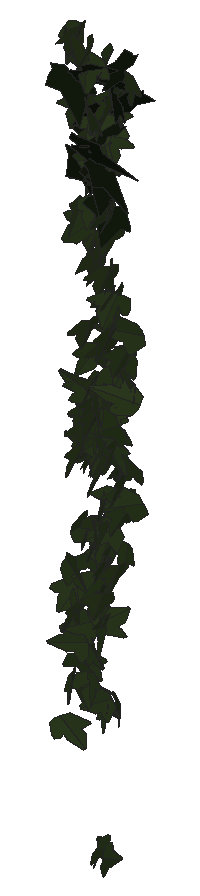
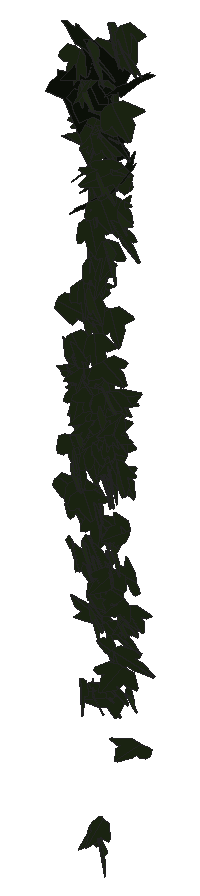
# SketchUp Ruby script. Lengths in inches.
U = 1.inch
M = Sketchup.active_model
def pt(a) = Geom::Point3d.new(a.map { |v| v * U })
def face(e, loops, mat)
  f = e.add_face(loops[0].map { |a| pt(a) })
  loops[1..].each { |l| e.add_face(l.map { |a| pt(a) }).erase! }
  f.material = f.back_material = mat if mat
  f
end
# faces: each face lists its corners as indices into pts; further lists are holes
def faces(e, pts, list, mat = nil) = list.each { |f| face(e, (f[0].is_a?(Array) ? f : [f]).map { |l| l.map { |i| pts[i] } }, mat) }
# xy, xz, yz: faces in a plane at the given z, y or x. An outline is a flat list of corners, or four numbers for a rectangle; further outlines are holes
def ring(l) = l.size == 4 ? [[l[0], l[1]], [l[2], l[1]], [l[2], l[3]], [l[0], l[3]]] : l.each_slice(2).to_a
def flat(e, list, mat, &to3) = list.each { |f| face(e, (f[0].is_a?(Array) ? f : [f]).map { |l| ring(l).map { |u, v| to3.(u, v) } }, mat) }
def xy(e, z, list, mat = nil) = flat(e, list, mat) { |x, y| [x, y, z] }
def xz(e, y, list, mat = nil) = flat(e, list, mat) { |x, z| [x, y, z] }
def yz(e, x, list, mat = nil) = flat(e, list, mat) { |y, z| [x, y, z] }
def lines(e, pts, list) = list.each { |a, b| e.add_line(pt(pts[a]), pt(pts[b])) }
# prism: a flat outline (further loops are holes) pulled along v
def prism(e, loops, v, mat = nil)
  f = face(e, loops, mat); d = Geom::Vector3d.new(v.map { |x| x * U })
  f.pushpull(f.normal.samedirection?(d) ? d.length : -d.length)
end
def box(e, o, s, mat = nil) = prism(e, [[o, [o[0] + s[0], o[1], o[2]], [o[0] + s[0], o[1] + s[1], o[2]], [o[0], o[1] + s[1], o[2]]]], [0, 0, s[2]], mat)
def at(x, y, z, deg = 0) = Geom::Transformation.translation(pt([x, y, z])) * Geom::Transformation.rotation(ORIGIN, Z_AXIS, deg.degrees)
def axes(o, x, y, z) = Geom::Transformation.new([*x, 0, *y, 0, *z, 0, *pt(o).to_a, 1])
def part(name) = M.definitions.add(name)
# library, detail: a bought-in or finely detailed component or shape, given as its bounding box
def library(name, o, s) = part(name).tap { |d| box(d.entities, o, s) }
def detail(e, o, s) = box(e.add_group.entities, o, s)
def put(e, d, t, mat = nil) = e.add_instance(d, t).tap { |i| i.material = mat if mat }
def group(e, t, mat = nil) = e.add_group.tap { |g| g.transformation = t; g.material = mat if mat }.entities
root = M.entities
M.materials.add("1026 AP 7946 SUNNY SIDE UP").color = [254, 231, 186]
M.materials.add("efeu1").color = [18, 25, 13]
M.materials.add("efeu2").color = [43, 57, 29]
c1 = part("ivyleaf_10")
p = [[0,0.5,-0.03],[-0.0625,2.02,-0.43],[-0.19,2.01,-0.46],[-0.54,1.05,-0.29],[-0.52,0.625,-0.18],[-0.83,0.76,-0.28],
  [-1.16,0.64,-0.33],[-1.15,0.33,-0.24],[-0.77,-0.39,0.02],[-0.3,-0.51,0.16],[0.04,-0.48,0.23],[-0.02,2.01,-0.4375],
  [-0.06,2.01,-0.43],[0.04,-0.49,0.23],[0.67,-0.49,0.14],[1.38,0.36,-0.2],[1.375,0.51,-0.24],[0.81,0.65,-0.19],
  [0.62,0.59,-0.15],[0.6,1.09,-0.28],[0.5,1.23,-0.31]]
faces(c1.entities,p,[[0,1,2,3,4,5,6,7,8,9,10],[11,12,0,13,14,15,16,17,18,19,20]],"efeu2")
c2 = part("ivyleaf_9")
p = [[1.54,2.16,1.25],[1.36,2.04,1.19],[-0.21,0.99,0.68],[-0.71,1.11,0.82],[-0.85,0.86,0.67],[-0.8,0.17,0.21],
  [-0.9,-0.01,0.1],[-0.67,-0.16,-0.02],[-0.08,-0.08,-0.05],[-0.03,-0.6,-0.4],[0.65,-0.88,-0.66],[0.83,-0.6,-0.49],
  [1.29,-0.42,-0.43],[1.8125,-0.07,-0.26],[1.21,0.44,0.15]]
faces(c2.entities,p,[[0,1,2,3,4,5,6,7,8,9,10,11,12,13,14]],"efeu1")
put(root,c1,axes([96.59,212.76,256.66],[0.16528,-0.03339,-0.18493],[-0.28245,0.01701,-0.11164],[0.04984,0.20716,-0.01939]),"1026 AP 7946 SUNNY SIDE UP")
put(root,c1,axes([96.42,212.9375,259.95],[0.03193,-0.19079,0.09635],[0.02892,-0.09312,-0.19805],[0.33361,0.02633,0.00795]),"1026 AP 7946 SUNNY SIDE UP")
put(root,c1,axes([96.55,212.97,260.11],[-0.3057,0.02603,0.089],[-0.13977,-0.02208,-0.19969],[-0.02302,-0.21154,0.03053]),"1026 AP 7946 SUNNY SIDE UP")
put(root,c1,axes([96.36,212.93,267.5],[0.28838,-0.15534,0.08831],[0.07617,-0.07607,-0.24669],[0.26908,0.18802,-0.02482]),"1026 AP 7946 SUNNY SIDE UP")
put(root,c1,axes([96.45,212.8,257.53],[0.30391,0.0384,-0.06901],[-0.09836,-0.02901,-0.20255],[-0.0717,0.20256,-0.01467]),"1026 AP 7946 SUNNY SIDE UP")
put(root,c1,axes([96.3125,212.73,255.11],[0.20943,0.10817,0.11767],[0.1516,0.06111,-0.17603],[-0.19457,0.16404,-0.0105]),"1026 AP 7946 SUNNY SIDE UP")
put(root,c1,axes([96.55,212.71,267.67],[-0.02234,-0.25481,-0.00265],[0.00583,0.00092,-0.26288],[0.40063,-0.01422,0.00368]),"1026 AP 7946 SUNNY SIDE UP")
put(root,c1,axes([96.61,212.87,266.35],[-0.1677,-0.21279,0.08333],[-0.02614,-0.08313,-0.24472],[0.35767,-0.10584,0.02118]),"1026 AP 7946 SUNNY SIDE UP")
put(root,c1,axes([96.59,212.95,260.78],[-0.04227,-0.2068,0.07166],[-0.00557,-0.07084,-0.21519],[0.34363,-0.02659,0.00533]),"1026 AP 7946 SUNNY SIDE UP")
put(root,c1,axes([96.59,212.92,260.48],[-0.10699,-0.20863,-0.01607],[0.01691,0.01165,-0.22591],[0.3284,-0.06857,0.00639]),"1026 AP 7946 SUNNY SIDE UP")
put(root,c1,axes([96.56,212.68,257.3],[0.05615,-0.02915,-0.22101],[0.02756,0.21694,-0.02611],[0.33905,-0.01281,0.03872]),"1026 AP 7946 SUNNY SIDE UP")
put(root,c1,axes([96.8,212.81,261.16],[-0.18364,-0.02128,-0.19752],[-0.30314,0.01117,0.11984],[-0.00232,0.22412,-0.0234]),"1026 AP 7946 SUNNY SIDE UP")
put(root,c1,axes([96.45,212.73,255.99],[0.12305,-0.09537,0.17263],[0.15601,-0.13583,-0.12776],[0.26082,0.12624,-0.00503]),"1026 AP 7946 SUNNY SIDE UP")
put(root,c1,axes([96.55,212.63,267.52],[-0.30771,0.1632,-0.02854],[0.00764,-0.0378,-0.26029],[-0.28121,-0.1796,0.02416]),"1026 AP 7946 SUNNY SIDE UP")
put(root,c1,axes([96.59,213,259.97],[0.09491,-0.20168,-0.03352],[-0.00023,0.03269,-0.21648],[0.32095,0.05966,0.00975]),"1026 AP 7946 SUNNY SIDE UP")
put(root,c1,axes([96.59,212.7,257.29],[0.04855,-0.17441,0.10361],[0.01151,-0.10171,-0.18282],[0.31714,0.03039,-0.00923]),"1026 AP 7946 SUNNY SIDE UP")
put(root,c1,axes([96.6875,212.73,264.2],[0.27516,-0.13573,-0.11826],[-0.15734,0.05663,-0.22731],[0.23009,0.20104,-0.01401]),"1026 AP 7946 SUNNY SIDE UP")
put(root,c1,axes([96.73,212.99,260.65],[-0.28813,-0.05134,-0.10827],[-0.1693,-0.00089,0.19439],[-0.0708,0.2111,-0.0242]),"1026 AP 7946 SUNNY SIDE UP")
put(root,c1,axes([96.54,212.99,260.87],[0.01949,0.21668,-0.02469],[-0.00003,-0.02523,-0.22373],[-0.34301,0.01231,-0.00138]),"1026 AP 7946 SUNNY SIDE UP")
put(root,c2,axes([96.49,212.91,265.16],[0.17587,-0.14957,-0.16549],[0.16614,-0.12026,0.19145],[-0.3014,-0.15356,0.00896]),"1026 AP 7946 SUNNY SIDE UP")
put(root,c1,axes([96.75,212.74,257.07],[0.21043,-0.06874,-0.15313],[-0.22571,0.04213,-0.15336],[0.12281,0.19522,-0.01948]),"1026 AP 7946 SUNNY SIDE UP")
put(root,c2,axes([96.48,212.69,266.83],[-0.02459,-0.25041,-0.01019],[0.00763,0.00819,-0.25839],[0.3939,-0.01579,0.00437]),"1026 AP 7946 SUNNY SIDE UP")
put(root,c1,axes([96.63,212.92,258.62],[0.11432,-0.191,-0.02471],[-0.00597,0.02306,-0.21035],[0.30242,0.07266,0.00519]),"1026 AP 7946 SUNNY SIDE UP")
put(root,c1,axes([96.5625,212.76,264.5],[0.08499,-0.1559,0.17875],[0.11831,-0.15789,-0.17036],[0.34827,0.09168,0.01425]),"1026 AP 7946 SUNNY SIDE UP")
put(root,c1,axes([96.71,212.9,261.22],[-0.25836,-0.13814,0.06274],[-0.02668,-0.07367,-0.21694],[0.23638,-0.1593,0.04409]),"1026 AP 7946 SUNNY SIDE UP")
put(root,c1,axes([96.67,213.03,259.88],[0.12107,-0.18948,-0.05398],[-0.00487,0.05395,-0.20967],[0.30864,0.07518,0.01787]),"1026 AP 7946 SUNNY SIDE UP")
put(root,c1,axes([96.56,212.88,257.67],[-0.27039,0.04284,-0.10368],[0.14124,-0.05246,-0.181],[-0.09875,-0.19234,0.02501]),"1026 AP 7946 SUNNY SIDE UP")
put(root,c1,axes([96.72,212.96,261.84],[0.16955,0.15754,-0.11644],[-0.14754,-0.07192,-0.19438],[-0.26773,0.1394,0.03338]),"1026 AP 7946 SUNNY SIDE UP")
put(root,c1,axes([96.43,212.67,258.01],[0.09325,-0.03481,0.22212],[0.31671,-0.07819,-0.07047],[0.13357,0.20971,0.01203]),"1026 AP 7946 SUNNY SIDE UP")
put(root,c1,axes([96.625,212.97,260.16],[0.00381,0.20896,-0.05279],[-0.00198,-0.05241,-0.21559],[-0.33874,0.00266,0.00067]),"1026 AP 7946 SUNNY SIDE UP")
put(root,c1,axes([96.67,212.62,258.76],[0.03395,-0.02797,0.23445],[-0.05757,0.22539,0.03342],[-0.35616,-0.0391,0.01695]),"1026 AP 7946 SUNNY SIDE UP")
put(root,c1,axes([96.62,212.79,256.36],[-0.26873,-0.07694,-0.09459],[0.141,0.02276,-0.19238],[0.12411,-0.19246,0.01375]),"1026 AP 7946 SUNNY SIDE UP")
put(root,c1,axes([96.74,212.9,263.83],[0.12556,-0.21826,-0.05346],[-0.02461,0.04821,-0.23913],[0.35145,0.08135,0.00236]),"1026 AP 7946 SUNNY SIDE UP")
put(root,c1,axes([96.73,212.89,258.39],[0.10867,-0.17815,-0.07354],[-0.01647,0.07119,-0.19583],[0.30074,0.06827,0.01585]),"1026 AP 7946 SUNNY SIDE UP")
put(root,c1,axes([96.72,212.94,261.34],[0.14003,-0.1976,0.05569],[0.01546,-0.05597,-0.22317],[0.32222,0.08856,-0.01349]),"1026 AP 7946 SUNNY SIDE UP")
put(root,c1,axes([96.77,212.93,261],[0.00581,-0.21472,0.0594],[-0.00322,-0.05891,-0.22156],[0.35007,0.00302,-0.00302]),"1026 AP 7946 SUNNY SIDE UP")
put(root,c1,axes([96.64,212.9375,258.13],[-0.15915,-0.12646,-0.13155],[0.17791,0.068,-0.16227],[0.21852,-0.14746,0.0363]),"1026 AP 7946 SUNNY SIDE UP")
put(root,c1,axes([96.77,212.96,260.5],[-0.33745,-0.00833,-0.00268],[0.00752,-0.06006,-0.21274],[0.01145,-0.20605,0.0608]),"1026 AP 7946 SUNNY SIDE UP")
put(root,c1,axes([96.58,212.91,265.33],[-0.18912,-0.09021,-0.20199],[0.27353,0.09136,-0.1531],[0.19964,-0.21063,0.01841]),"1026 AP 7946 SUNNY SIDE UP")
put(root,c1,axes([96.82,212.92,265.19],[0.06552,-0.23859,0.0421],[0.00101,-0.04274,-0.24967],[0.38098,0.04115,-0.00658]),"1026 AP 7946 SUNNY SIDE UP")
put(root,c1,axes([96.68,212.9,265.21],[0.3265,0.11157,0.0753],[0.08463,0.05238,-0.24168],[-0.19129,0.2136,0.0216]),"1026 AP 7946 SUNNY SIDE UP")
put(root,c1,axes([96.85,212.92,265.91],[-0.04209,-0.23527,0.0793],[0.00131,-0.07885,-0.24422],[0.3899,-0.02513,0.00938]),"1026 AP 7946 SUNNY SIDE UP")
put(root,c1,axes([96.85,212.64,262.52],[-0.05945,-0.22787,0.00666],[0.00455,-0.00835,-0.23796],[0.35848,-0.03768,0.00412]),"1026 AP 7946 SUNNY SIDE UP")
put(root,c1,axes([96.85,212.66,267.27],[-0.3823,0.0869,-0.03679],[-0.01893,-0.11637,-0.2309],[-0.15822,-0.19605,0.11651]),"1026 AP 7946 SUNNY SIDE UP")
put(root,c1,axes([96.88,212.79,257.86],[-0.14831,-0.1418,0.12037],[-0.02439,-0.12559,-0.16948],[0.28869,-0.08346,0.04752]),"1026 AP 7946 SUNNY SIDE UP")
put(root,c1,axes([96.85,212.96,260.36],[-0.00106,-0.1401,0.16872],[-0.00337,-0.16456,-0.14529],[0.33982,-0.00207,-0.00091]),"1026 AP 7946 SUNNY SIDE UP")
put(root,c1,axes([96.91,212.57,267.53],[0.07247,-0.22036,-0.10877],[-0.04331,0.09558,-0.23887],[0.4076,0.04934,-0.00604]),"1026 AP 7946 SUNNY SIDE UP")
put(root,c1,axes([96.88,212.81,259.71],[0.10536,-0.20043,-0.02333],[-0.0227,0.01783,-0.21746],[0.31615,0.06808,-0.00784]),"1026 AP 7946 SUNNY SIDE UP")
put(root,c1,axes([96.89,212.85,264.6],[-0.21488,-0.18704,0.07108],[0.01551,-0.09111,-0.23128],[0.31367,-0.12363,0.06013]),"1026 AP 7946 SUNNY SIDE UP")
put(root,c1,axes([96.74,212.75,256.04],[0.26852,-0.07153,0.10281],[0.13814,-0.04924,-0.19074],[0.13562,0.19178,-0.00927]),"1026 AP 7946 SUNNY SIDE UP")
put(root,c1,axes([96.91,212.96,259.21],[0.1288,-0.17862,-0.07762],[-0.02735,0.07359,-0.2015],[0.30297,0.08258,0.01481]),"1026 AP 7946 SUNNY SIDE UP")
put(root,c2,axes([97.14,212.72,265.97],[-0.11502,0.21182,0.07801],[-0.15054,0.04167,-0.22595],[-0.34756,-0.08815,0.07205]),"1026 AP 7946 SUNNY SIDE UP")
put(root,c1,axes([96.88,212.85,263.49],[0.01975,-0.2134,-0.10548],[0.06535,0.10174,-0.21514],[0.36555,-0.00666,0.04416]),"1026 AP 7946 SUNNY SIDE UP")
put(root,c1,axes([96.875,212.96,260.57],[0.08177,0.17841,-0.11614],[-0.03426,-0.112,-0.19188],[-0.33093,0.05568,-0.00883]),"1026 AP 7946 SUNNY SIDE UP")
put(root,c1,axes([96.9,212.68,263.74],[-0.0642,-0.2095,-0.10787],[0.06837,0.09644,-0.21818],[0.36103,-0.05552,0.02213]),"1026 AP 7946 SUNNY SIDE UP")
put(root,c1,axes([96.91,212.97,261.24],[-0.30803,-0.0968,-0.03494],[0.06303,-0.00622,-0.22389],[0.14814,-0.19862,0.0226]),"1026 AP 7946 SUNNY SIDE UP")
put(root,c1,axes([97,212.49,266.47],[-0.27182,0.16744,0.09835],[-0.12881,0.05114,-0.24655],[-0.2956,-0.17626,0.017]),"1026 AP 7946 SUNNY SIDE UP")
put(root,c1,axes([96.96,212.82,258.92],[-0.23151,-0.1477,-0.01816],[0.03091,0.00407,-0.21453],[0.23169,-0.14813,0.01048]),"1026 AP 7946 SUNNY SIDE UP")
put(root,c1,axes([96.97,212.66,260.93],[0.01742,-0.21513,0.06245],[0.01115,-0.06155,-0.22224],[0.35179,0.0126,0.00395]),"1026 AP 7946 SUNNY SIDE UP")
put(root,c1,axes([96.95,212.9375,260.58],[-0.30065,0.09682,-0.02147],[0.01287,-0.03091,-0.21961],[-0.15538,-0.1899,0.02336]),"1026 AP 7946 SUNNY SIDE UP")
put(root,c1,axes([96.9375,212.88,266.1],[0.2824,0.15726,-0.0784],[-0.06367,-0.07001,-0.24501],[-0.26786,0.18243,-0.02442]),"1026 AP 7946 SUNNY SIDE UP")
put(root,c1,axes([96.98,212.86,258.15],[0.07507,-0.2004,0.00763],[-0.00297,-0.00923,-0.21225],[0.31539,0.04761,-0.00381]),"1026 AP 7946 SUNNY SIDE UP")
put(root,c1,axes([96.99,212.9,260.1875],[-0.09526,-0.18422,0.10269],[0.01705,-0.10744,-0.19634],[0.3297,-0.04767,0.03982]),"1026 AP 7946 SUNNY SIDE UP")
put(root,c1,axes([97.01,212.95,260.13],[-0.13687,-0.19343,0.01376],[0.00209,-0.01644,-0.21846],[0.30498,-0.08669,0.00767]),"1026 AP 7946 SUNNY SIDE UP")
put(root,c2,axes([97.13,212.91,266.51],[-0.11429,0.16948,-0.17714],[-0.00896,-0.18168,-0.18205],[-0.3806,-0.04662,0.05748]),"1026 AP 7946 SUNNY SIDE UP")
put(root,c1,axes([96.82,212.84,258.71],[0.02982,-0.0363,0.21506],[0.22398,-0.15326,-0.04164],[0.24709,0.14331,0.0118]),"1026 AP 7946 SUNNY SIDE UP")
put(root,c1,axes([97.01,212.73,253.1],[0.10064,-0.17295,-0.09948],[-0.03115,0.09435,-0.18899],[0.30915,0.06581,0.01334]),"1026 AP 7946 SUNNY SIDE UP")
put(root,c1,axes([97.02,212.92,262.98],[0.01441,-0.23294,0.02091],[-0.00004,-0.02164,-0.24028],[0.36785,0.00912,-0.00084]),"1026 AP 7946 SUNNY SIDE UP")
put(root,c1,axes([96.91,212.8,257.51],[-0.00238,-0.1981,-0.08195],[0.04326,-0.07795,0.20185],[-0.33221,-0.00873,0.02687]),"1026 AP 7946 SUNNY SIDE UP")
put(root,c1,axes([97.02,212.93,267.28],[0.15553,-0.23452,-0.00585],[-0.01049,0.0019,-0.26214],[0.36867,0.09899,-0.00499]),"1026 AP 7946 SUNNY SIDE UP")
put(root,c1,axes([96.99,212.78,260.36],[0.19866,-0.1712,0.03233],[0.01133,-0.0348,-0.21888],[0.27373,0.12569,-0.0144]),"1026 AP 7946 SUNNY SIDE UP")
put(root,c1,axes([97.02,212.85,262.1],[-0.07758,-0.2211,-0.0361],[0.01859,0.03197,-0.23315],[0.35121,-0.05053,0.00437]),"1026 AP 7946 SUNNY SIDE UP")
put(root,c1,axes([96.79,212.73,256.64],[0.05049,-0.02592,0.20407],[0.28065,-0.08674,-0.04198],[0.14163,0.18112,0.01043]),"1026 AP 7946 SUNNY SIDE UP")
put(root,c1,axes([97.14,212.6875,255.83],[0.21874,-0.08832,-0.14132],[-0.20228,0.05044,-0.16817],[0.15671,0.18838,-0.0198]),"1026 AP 7946 SUNNY SIDE UP")
put(root,c1,axes([96.95,212.9,265.86],[-0.00619,0.24826,-0.02509],[0.00316,-0.02573,-0.25593],[-0.39244,-0.00412,-0.00166]),"1026 AP 7946 SUNNY SIDE UP")
put(root,c1,axes([96.8125,212.74,255.83],[-0.19346,0.00776,-0.17627],[0.26283,-0.0408,-0.12593],[-0.05911,-0.2068,0.01697]),"1026 AP 7946 SUNNY SIDE UP")
put(root,c1,axes([97.03,212.86,258.21],[0.15582,-0.17188,-0.06029],[-0.02383,0.0575,-0.20348],[0.28402,0.09912,0.016]),"1026 AP 7946 SUNNY SIDE UP")
put(root,c1,axes([97.01,212.71,261.21],[-0.03687,0.22084,-0.00624],[-0.05068,-0.01069,-0.22629],[-0.34373,-0.02211,0.03404]),"1026 AP 7946 SUNNY SIDE UP")
put(root,c1,axes([96.89,212.92,265.76],[0.33101,0.11747,0.06735],[0.0777,0.04402,-0.24768],[-0.19604,0.21579,0.01555]),"1026 AP 7946 SUNNY SIDE UP")
put(root,c1,axes([96.94,212.92,266.15],[0.17947,0.20789,0.08586],[0.00643,0.09029,-0.24069],[-0.35143,0.10782,0.03944]),"1026 AP 7946 SUNNY SIDE UP")
put(root,c1,axes([96.98,212.91,258.51],[0.27049,-0.11339,0.02637],[0.02408,-0.02437,-0.21205],[0.18142,0.1723,-0.01118]),"1026 AP 7946 SUNNY SIDE UP")
put(root,c1,axes([97.0625,212.85,263.45],[-0.08214,-0.2274,0.03717],[0.00374,-0.03885,-0.24033],[0.36234,-0.05115,0.01091]),"1026 AP 7946 SUNNY SIDE UP")
put(root,c2,axes([96.93,212.92,265.03],[-0.03914,-0.20993,0.12522],[0.00402,-0.1236,-0.21797],[0.38235,-0.02019,0.01511]),"1026 AP 7946 SUNNY SIDE UP")
put(root,c1,axes([97.09,212.875,264.15],[-0.13786,-0.22269,0.01114],[0.0029,-0.0137,-0.24653],[0.35066,-0.08744,0.00642]),"1026 AP 7946 SUNNY SIDE UP")
put(root,c2,axes([96.72,212.64,265.66],[0.30064,-0.06927,0.15389],[0.21179,-0.06692,-0.20941],[0.1499,0.23347,-0.01277]),"1026 AP 7946 SUNNY SIDE UP")
put(root,c1,axes([97.07,212.73,259.33],[0.11078,-0.19048,-0.05133],[-0.00488,0.0507,-0.20842],[0.30913,0.06906,0.01511]),"1026 AP 7946 SUNNY SIDE UP")
put(root,c1,axes([97,212.97,260.73],[0.05998,0.21408,-0.0099],[0.00711,-0.0118,-0.22398],[-0.33697,0.03786,-0.00649]),"1026 AP 7946 SUNNY SIDE UP")
put(root,c1,axes([97.1,212.65,257.67],[-0.13027,-0.18786,0.03005],[-0.00619,-0.03127,-0.2115],[0.29912,-0.08246,0.00871]),"1026 AP 7946 SUNNY SIDE UP")
put(root,c1,axes([97.19,212.78,258.875],[0.24918,-0.06087,-0.13816],[-0.21035,0.02169,-0.17331],[0.09566,0.20624,-0.02123]),"1026 AP 7946 SUNNY SIDE UP")
put(root,c2,axes([96.83,212.62,267.06],[0.355,0.07897,0.10058],[0.15067,0.02793,-0.23887],[-0.14196,0.22713,-0.002]),"1026 AP 7946 SUNNY SIDE UP")
put(root,c1,axes([97.11,212.8125,261.22],[-0.34837,-0.01665,0.01194],[-0.01579,-0.02157,-0.22802],[0.02782,-0.22081,0.02007]),"1026 AP 7946 SUNNY SIDE UP")
put(root,c1,axes([97.11,213.01,259.39],[-0.2174,-0.14537,0.05711],[0.00834,-0.07955,-0.19878],[0.24496,-0.12631,0.05745]),"1026 AP 7946 SUNNY SIDE UP")
put(root,c1,axes([97.03,212.97,260.87],[0.0948,0.2108,-0.0141],[-0.00454,-0.01465,-0.22596],[-0.33226,0.06034,-0.00093]),"1026 AP 7946 SUNNY SIDE UP")
put(root,c1,axes([97.1,212.97,258.47],[0.14946,-0.17506,-0.04973],[-0.00066,0.05317,-0.20337],[0.28513,0.09188,0.0256]),"1026 AP 7946 SUNNY SIDE UP")
put(root,c1,axes([97.11,212.96,258.49],[0.07129,-0.19334,0.05222],[0.00554,-0.05232,-0.20472],[0.31468,0.04472,-0.00822]),"1026 AP 7946 SUNNY SIDE UP")
put(root,c1,axes([97.07,212.96,261.56],[0.16088,0.19443,0.03361],[-0.04106,0.0486,-0.2212],[-0.30698,0.09539,0.0472]),"1026 AP 7946 SUNNY SIDE UP")
put(root,c1,axes([97.15,212.9,266.58],[-0.02585,-0.20729,0.14762],[0.01134,-0.1451,-0.21449],[0.39713,-0.00935,0.01573]),"1026 AP 7946 SUNNY SIDE UP")
put(root,c1,axes([97.09,212.85,261.31],[-0.17672,0.18968,-0.03564],[0.00793,-0.03838,-0.22683],[-0.30338,-0.1115,0.01483]),"1026 AP 7946 SUNNY SIDE UP")
put(root,c1,axes([97.16,212.71,257.31],[0.03337,-0.2048,0.01577],[0.0006,-0.01652,-0.2122],[0.32307,0.02119,-0.00124]),"1026 AP 7946 SUNNY SIDE UP")
put(root,c2,axes([96.98,212.76,265.35],[0.162,-0.20644,-0.08536],[-0.04219,0.07781,-0.237],[0.34653,0.10598,0.01105]),"1026 AP 7946 SUNNY SIDE UP")
put(root,c1,axes([97.36,212.6875,260.82],[-0.21721,0.06598,0.17838],[-0.28004,0.0107,-0.15084],[-0.07843,-0.22095,0.04456]),"1026 AP 7946 SUNNY SIDE UP")
put(root,c1,axes([97.05,212.73,257.27],[-0.01987,-0.07218,-0.19805],[0.08103,-0.18715,0.06795],[-0.31194,-0.04401,0.03027]),"1026 AP 7946 SUNNY SIDE UP")
put(root,c1,axes([97.16,212.69,264.63],[0.01745,-0.23514,-0.05853],[0.02563,0.05614,-0.24143],[0.37901,0.00703,0.01902]),"1026 AP 7946 SUNNY SIDE UP")
put(root,c2,axes([97.11,212.91,264.58],[-0.10391,-0.21932,0.07868],[-0.0226,-0.07669,-0.23628],[0.36512,-0.06716,0.00777]),"1026 AP 7946 SUNNY SIDE UP")
put(root,c1,axes([97.14,212.91,261.23],[0.34798,-0.00214,-0.01737],[-0.02661,-0.00916,-0.22785],[0.00227,0.22176,-0.00828]),"1026 AP 7946 SUNNY SIDE UP")
put(root,c1,axes([97.18,212.92,263.05],[0.00285,-0.22937,-0.04893],[0.02935,0.04618,-0.23525],[0.36674,-0.00191,0.01921]),"1026 AP 7946 SUNNY SIDE UP")
put(root,c1,axes([97.16,212.82,258.05],[0.16965,-0.16986,0.04178],[0.04008,-0.03298,-0.20746],[0.27202,0.1108,0.00451]),"1026 AP 7946 SUNNY SIDE UP")
put(root,c1,axes([97.15,212.91,266.6],[0.11977,-0.18913,0.15385],[0.07226,-0.1435,-0.21069],[0.37304,0.08852,-0.00859]),"1026 AP 7946 SUNNY SIDE UP")
put(root,c1,axes([97.11,212.72,258.85],[0.07264,-0.0965,0.18941],[0.12262,-0.16711,-0.11119],[0.30343,0.09063,-0.00041]),"1026 AP 7946 SUNNY SIDE UP")
put(root,c1,axes([97.11,212.7,257.03],[0.04981,-0.12925,0.15987],[0.1334,-0.13483,-0.13369],[0.28915,0.08446,0.03414]),"1026 AP 7946 SUNNY SIDE UP")
put(root,c1,axes([97.19,212.79,263.51],[0.10958,-0.20642,-0.09871],[0.02233,0.10277,-0.21953],[0.35636,0.05703,0.04411]),"1026 AP 7946 SUNNY SIDE UP")
put(root,c1,axes([97.24,212.82,263],[-0.20836,-0.16906,0.09496],[0.01282,-0.11778,-0.20897],[0.30323,-0.11119,0.07409]),"1026 AP 7946 SUNNY SIDE UP")
put(root,c1,axes([97.23,213.01,259.97],[0.01648,-0.207,-0.04718],[-0.00121,0.04464,-0.21325],[0.33296,0.01041,0.00156]),"1026 AP 7946 SUNNY SIDE UP")
put(root,c1,axes([97.24,212.7,262.46],[0.01488,-0.23146,0.06004],[0.0001,-0.05963,-0.23899],[0.37582,0.00918,-0.00231]),"1026 AP 7946 SUNNY SIDE UP")
put(root,c1,axes([97.16,212.91,266.66],[-0.08559,0.24662,-0.02551],[0.00281,-0.0264,-0.26031],[-0.38996,-0.05432,0.00372]),"1026 AP 7946 SUNNY SIDE UP")
put(root,c1,axes([97.24,212.79,260.71],[-0.32131,0.07392,0.00021],[-0.01385,-0.02497,-0.22234],[-0.11541,-0.20281,0.02609]),"1026 AP 7946 SUNNY SIDE UP")
put(root,c1,axes([97.22,212.97,261.18],[-0.13714,-0.18481,-0.08909],[0.06413,0.0752,-0.21003],[0.31365,-0.09618,0.00399]),"1026 AP 7946 SUNNY SIDE UP")
put(root,c1,axes([97.03,212.77,257.17],[0.25419,-0.02585,-0.14393],[0.22311,0.02396,0.16488],[-0.00577,-0.21222,0.03487]),"1026 AP 7946 SUNNY SIDE UP")
put(root,c2,axes([97.28,212.9,266.62],[0.16,0.22615,-0.05337],[-0.01582,-0.05362,-0.25546],[-0.36492,0.10148,-0.01232]),"1026 AP 7946 SUNNY SIDE UP")
put(root,c1,axes([97.125,212.72,255.7],[0.14323,-0.08747,0.16288],[0.1639,-0.11987,-0.13048],[0.23291,0.13814,-0.00835]),"1026 AP 7946 SUNNY SIDE UP")
put(root,c1,axes([97.22,212.48,253.29],[-0.04148,-0.1272,-0.1611],[0.07614,0.14834,-0.13247],[0.30677,-0.05402,0.0111]),"1026 AP 7946 SUNNY SIDE UP")
put(root,c1,axes([97.28,212.99,260.04],[0.05128,-0.20756,-0.04134],[0.00064,0.03947,-0.21612],[0.33207,0.03198,0.0068]),"1026 AP 7946 SUNNY SIDE UP")
put(root,c1,axes([97.16,212.74,260.41],[-0.28132,0.03739,-0.11768],[0.16028,-0.06205,-0.18541],[-0.10074,-0.20312,0.03364]),"1026 AP 7946 SUNNY SIDE UP")
put(root,c1,axes([97.3,212.97,259.47],[-0.11825,-0.19067,0.04861],[0.00802,-0.05355,-0.21005],[0.30917,-0.07154,0.02404]),"1026 AP 7946 SUNNY SIDE UP")
put(root,c1,axes([97.3,212.8,258.1875],[-0.05865,-0.20051,0.03064],[0.01062,-0.03261,-0.20991],[0.31883,-0.0358,0.01263]),"1026 AP 7946 SUNNY SIDE UP")
put(root,c1,axes([97.35,212.9375,262.05],[-0.09859,-0.20968,0.06444],[-0.00943,-0.06464,-0.22549],[0.34447,-0.06178,0.01227]),"1026 AP 7946 SUNNY SIDE UP")
put(root,c1,axes([97.32,212.86,260.49],[0.05081,-0.20006,0.07876],[0.01913,-0.07663,-0.20922],[0.33686,0.03453,0]),"1026 AP 7946 SUNNY SIDE UP")
put(root,c1,axes([97.36,212.69,262.8125],[0.13606,-0.21561,-0.06779],[-0.0402,0.05932,-0.23899],[0.35162,0.09022,-0.00109]),"1026 AP 7946 SUNNY SIDE UP")
put(root,c1,axes([97.375,212.55,264.79],[0.05661,-0.19415,-0.17256],[-0.04477,0.16395,-0.20245],[0.39956,0.04588,0.00176]),"1026 AP 7946 SUNNY SIDE UP")
put(root,c1,axes([97.32,212.96,259.77],[0.10362,-0.19529,0.10353],[0.03907,-0.09878,-0.21278],[0.34394,0.07006,-0.00702]),"1026 AP 7946 SUNNY SIDE UP")
put(root,c1,axes([97.38,212.9,259.1875],[-0.07117,-0.18147,0.0945],[-0.01392,-0.09318,-0.19279],[0.32015,-0.04439,0.01263]),"1026 AP 7946 SUNNY SIDE UP")
put(root,c1,axes([97.29,213.02,258.44],[0.25933,-0.11655,0.01521],[0.03527,0.00511,-0.20728],[0.18147,0.16557,0.01855]),"1026 AP 7946 SUNNY SIDE UP")
put(root,c2,axes([97.57,212.61,267.34],[-0.22024,0.21948,0.03553],[-0.05487,0.01705,-0.26733],[-0.34471,-0.14294,0.01985]),"1026 AP 7946 SUNNY SIDE UP")
put(root,c1,axes([97.34,212.96,261.44],[0.29038,-0.12494,0.00454],[-0.01394,-0.02218,-0.22857],[0.19613,0.18341,-0.02296]),"1026 AP 7946 SUNNY SIDE UP")
put(root,c1,axes([97.4,212.98,261.95],[0.25515,-0.13729,-0.07485],[-0.07496,0.0548,-0.21839],[0.23186,0.1688,0.01176]),"1026 AP 7946 SUNNY SIDE UP")
put(root,c1,axes([97.375,212.9,267.08],[-0.32025,0.15406,0.01054],[-0.03154,-0.01107,-0.26227],[-0.24063,-0.20359,0.02035]),"1026 AP 7946 SUNNY SIDE UP")
put(root,c1,axes([97.59,212.76,261.33],[0.01119,0.12492,0.19583],[-0.3009,-0.09847,0.07375],[0.19161,-0.16192,0.10437]),"1026 AP 7946 SUNNY SIDE UP")
put(root,c1,axes([97.39,212.72,255.8],[0.1508,-0.13056,-0.13865],[-0.02848,0.14323,-0.15647],[0.29262,0.08122,0.05622]),"1026 AP 7946 SUNNY SIDE UP")
put(root,c1,axes([97.62,212.8,262.54],[0.09819,-0.01307,-0.23258],[-0.35007,0.0371,-0.06546],[0.06172,0.23121,-0.00126]),"1026 AP 7946 SUNNY SIDE UP")
put(root,c1,axes([97.27,212.98,261.58],[-0.17918,0.14608,-0.1268],[0.10406,-0.10528,-0.19118],[-0.28266,-0.13136,0.01]),"1026 AP 7946 SUNNY SIDE UP")
put(root,c1,axes([97.6,212.89,259.42],[-0.17319,0.02402,0.18706],[-0.27084,-0.08521,-0.0966],[0.09731,-0.1944,0.06408]),"1026 AP 7946 SUNNY SIDE UP")
put(root,c2,axes([97.19,212.9,266.72],[0.11479,-0.07722,-0.23812],[0.30093,-0.13046,0.10662],[-0.23615,-0.20379,0.02012]),"1026 AP 7946 SUNNY SIDE UP")
put(root,c1,axes([97.53,212.83,260.14],[-0.28823,0.06165,0.11067],[-0.17405,0.00319,-0.19708],[-0.08632,-0.21226,0.02784]),"1026 AP 7946 SUNNY SIDE UP")
put(root,c1,axes([97.36,212.46,253.16],[0.01281,-0.09549,-0.192],[0.06972,0.18252,-0.09355],[0.32103,-0.03583,0.02798]),"1026 AP 7946 SUNNY SIDE UP")
